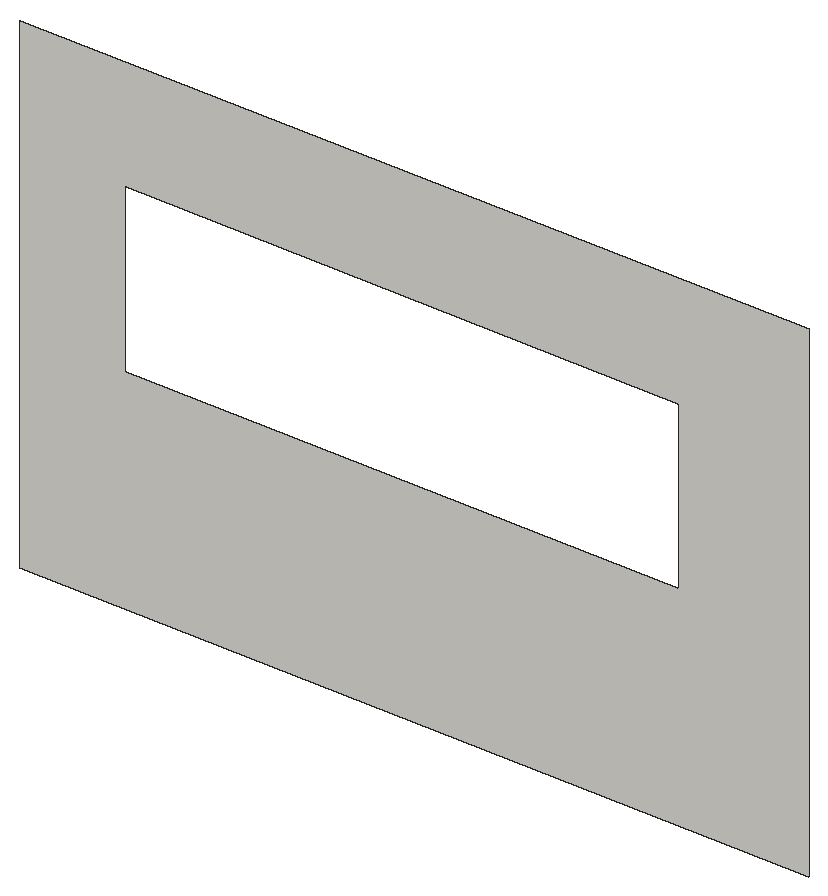
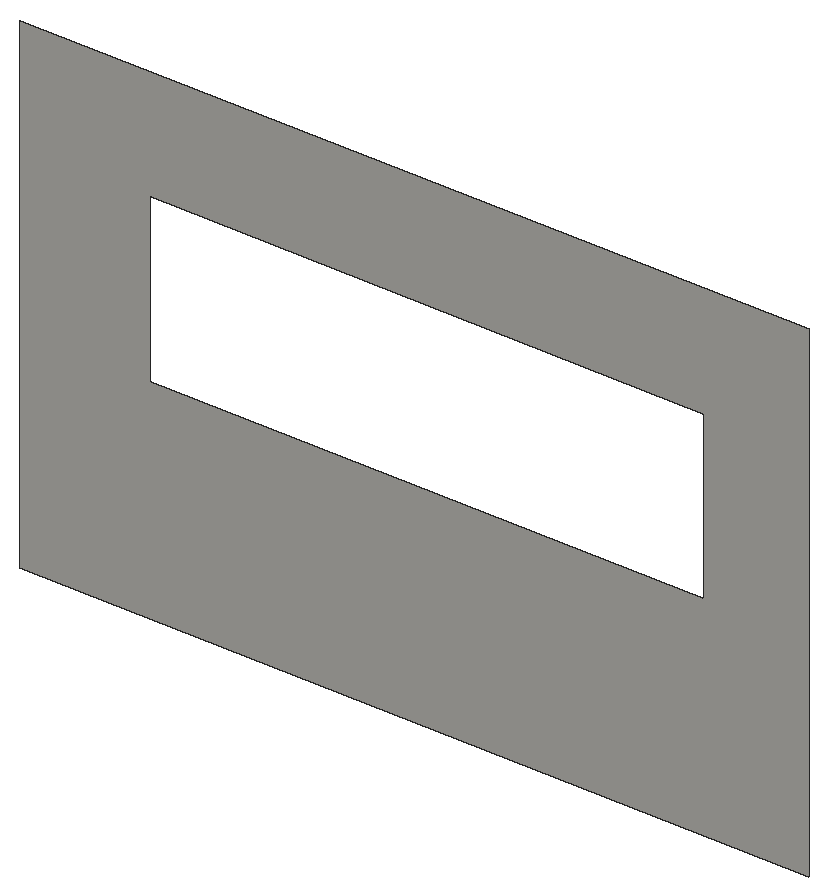
# SketchUp Ruby script. Lengths in inches.
U = 1.inch
M = Sketchup.active_model
def pt(a) = Geom::Point3d.new(a.map { |v| v * U })
def face(e, loops, mat)
  f = e.add_face(loops[0].map { |a| pt(a) })
  loops[1..].each { |l| e.add_face(l.map { |a| pt(a) }).erase! }
  f.material = f.back_material = mat if mat
  f
end
# faces: each face lists its corners as indices into pts; further lists are holes
def faces(e, pts, list, mat = nil) = list.each { |f| face(e, (f[0].is_a?(Array) ? f : [f]).map { |l| l.map { |i| pts[i] } }, mat) }
# xy, xz, yz: faces in a plane at the given z, y or x. An outline is a flat list of corners, or four numbers for a rectangle; further outlines are holes
def ring(l) = l.size == 4 ? [[l[0], l[1]], [l[2], l[1]], [l[2], l[3]], [l[0], l[3]]] : l.each_slice(2).to_a
def flat(e, list, mat, &to3) = list.each { |f| face(e, (f[0].is_a?(Array) ? f : [f]).map { |l| ring(l).map { |u, v| to3.(u, v) } }, mat) }
def xy(e, z, list, mat = nil) = flat(e, list, mat) { |x, y| [x, y, z] }
def xz(e, y, list, mat = nil) = flat(e, list, mat) { |x, z| [x, y, z] }
def yz(e, x, list, mat = nil) = flat(e, list, mat) { |y, z| [x, y, z] }
def lines(e, pts, list) = list.each { |a, b| e.add_line(pt(pts[a]), pt(pts[b])) }
# prism: a flat outline (further loops are holes) pulled along v
def prism(e, loops, v, mat = nil)
  f = face(e, loops, mat); d = Geom::Vector3d.new(v.map { |x| x * U })
  f.pushpull(f.normal.samedirection?(d) ? d.length : -d.length)
end
def box(e, o, s, mat = nil) = prism(e, [[o, [o[0] + s[0], o[1], o[2]], [o[0] + s[0], o[1] + s[1], o[2]], [o[0], o[1] + s[1], o[2]]]], [0, 0, s[2]], mat)
def at(x, y, z, deg = 0) = Geom::Transformation.translation(pt([x, y, z])) * Geom::Transformation.rotation(ORIGIN, Z_AXIS, deg.degrees)
def axes(o, x, y, z) = Geom::Transformation.new([*x, 0, *y, 0, *z, 0, *pt(o).to_a, 1])
def part(name) = M.definitions.add(name)
# library, detail: a bought-in or finely detailed component or shape, given as its bounding box
def library(name, o, s) = part(name).tap { |d| box(d.entities, o, s) }
def detail(e, o, s) = box(e.add_group.entities, o, s)
def put(e, d, t, mat = nil) = e.add_instance(d, t).tap { |i| i.material = mat if mat }
def group(e, t, mat = nil) = e.add_group.tap { |g| g.transformation = t; g.material = mat if mat }.entities
root = M.entities
M.materials.add("[Marble Carrara Gold Floor Tile]").color = [225, 223, 217]
xz(root,184.11,[[[321.5,0,469.67,92.125],[341.12,39.83,445.24,71.08]]],"[Marble Carrara Gold Floor Tile]")
